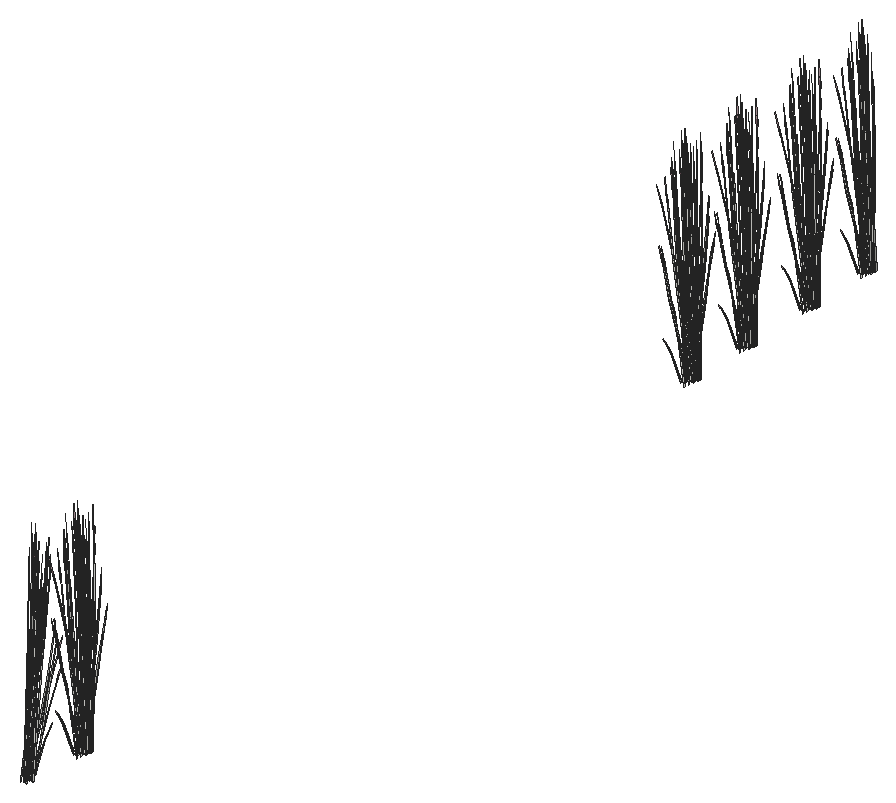
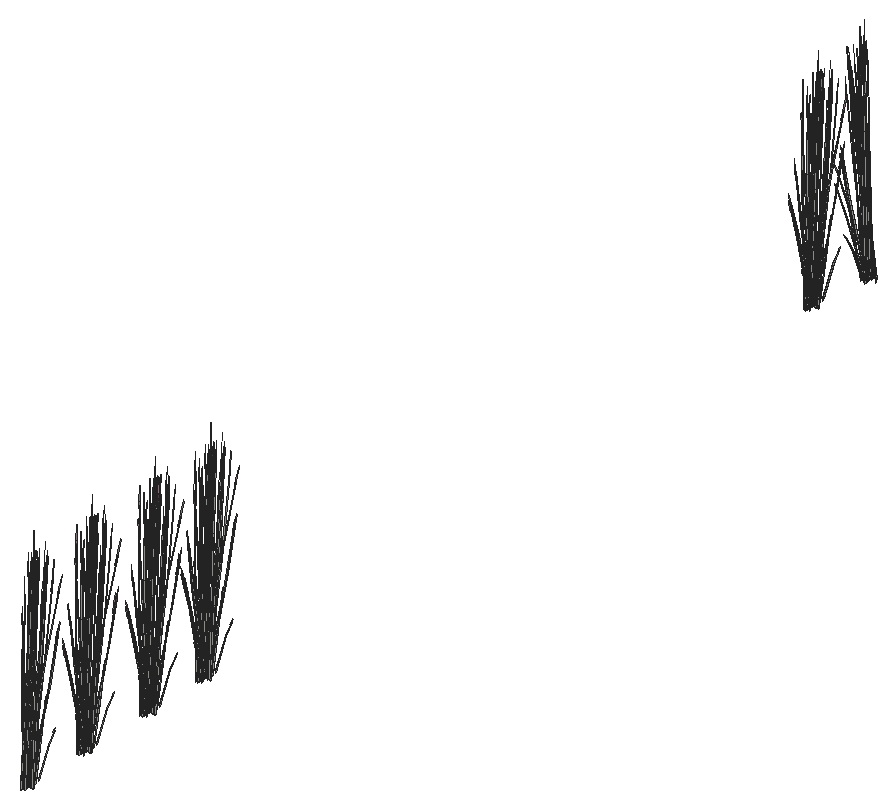
# SketchUp Ruby script. Lengths in inches.
U = 1.inch
M = Sketchup.active_model
def pt(a) = Geom::Point3d.new(a.map { |v| v * U })
def face(e, loops, mat)
  f = e.add_face(loops[0].map { |a| pt(a) })
  loops[1..].each { |l| e.add_face(l.map { |a| pt(a) }).erase! }
  f.material = f.back_material = mat if mat
  f
end
# faces: each face lists its corners as indices into pts; further lists are holes
def faces(e, pts, list, mat = nil) = list.each { |f| face(e, (f[0].is_a?(Array) ? f : [f]).map { |l| l.map { |i| pts[i] } }, mat) }
# xy, xz, yz: faces in a plane at the given z, y or x. An outline is a flat list of corners, or four numbers for a rectangle; further outlines are holes
def ring(l) = l.size == 4 ? [[l[0], l[1]], [l[2], l[1]], [l[2], l[3]], [l[0], l[3]]] : l.each_slice(2).to_a
def flat(e, list, mat, &to3) = list.each { |f| face(e, (f[0].is_a?(Array) ? f : [f]).map { |l| ring(l).map { |u, v| to3.(u, v) } }, mat) }
def xy(e, z, list, mat = nil) = flat(e, list, mat) { |x, y| [x, y, z] }
def xz(e, y, list, mat = nil) = flat(e, list, mat) { |x, z| [x, y, z] }
def yz(e, x, list, mat = nil) = flat(e, list, mat) { |y, z| [x, y, z] }
def lines(e, pts, list) = list.each { |a, b| e.add_line(pt(pts[a]), pt(pts[b])) }
# prism: a flat outline (further loops are holes) pulled along v
def prism(e, loops, v, mat = nil)
  f = face(e, loops, mat); d = Geom::Vector3d.new(v.map { |x| x * U })
  f.pushpull(f.normal.samedirection?(d) ? d.length : -d.length)
end
def box(e, o, s, mat = nil) = prism(e, [[o, [o[0] + s[0], o[1], o[2]], [o[0] + s[0], o[1] + s[1], o[2]], [o[0], o[1] + s[1], o[2]]]], [0, 0, s[2]], mat)
def at(x, y, z, deg = 0) = Geom::Transformation.translation(pt([x, y, z])) * Geom::Transformation.rotation(ORIGIN, Z_AXIS, deg.degrees)
def axes(o, x, y, z) = Geom::Transformation.new([*x, 0, *y, 0, *z, 0, *pt(o).to_a, 1])
def part(name) = M.definitions.add(name)
# library, detail: a bought-in or finely detailed component or shape, given as its bounding box
def library(name, o, s) = part(name).tap { |d| box(d.entities, o, s) }
def detail(e, o, s) = box(e.add_group.entities, o, s)
def put(e, d, t, mat = nil) = e.add_instance(d, t).tap { |i| i.material = mat if mat }
def group(e, t, mat = nil) = e.add_group.tap { |g| g.transformation = t; g.material = mat if mat }.entities
root = M.entities
M.materials.add("LightPink_Translucent").color = [144, 107, 117]
M.materials["LightPink_Translucent"].alpha = 0.75
c1 = part("blade")
p = [[2.15,0.21,22],[0,0.17,0],[0.09,0.45,0],[2.18,0.31,22],[2.29,0.31,22],[0.38,0.45,0],
  [2.48,0.24,33],[2.49,0.24,33],[2.48,0.22,33]]
faces(c1.entities,p,[[0,1,2,3],[4,5,2,3],[6,3,4,7],[8,0,3,6]])
c2 = part("seeds")
p = [[0.3,-0.1,1.38],[-0.01,-0.03,1.59],[-0.01,-0.03,0.03],[0.14,-0.07,-0.07],[0.29,-0.03,3],[0.15,0.01,3.11]]
faces(c2.entities,p,[[0,1,2,3],[1,0,4,5]],"LightPink_Translucent")
c3 = part("blade with seeds")
put(c3.entities,c1,at(0,0,0))
put(c3.entities,c2,axes([2.4,0.25,30.99],[1.5799,-0.05474,1.17369],[-0.12525,1.92788,0.29478],[-0.07173,-0.02425,1.56792]))
put(root,c3,axes([399.9,291.3,2.48],[-0.33032,-0.23318,0.49651],[0.19744,-0.41812,0],[0.07523,0.05311,1.57504]))
put(root,c3,axes([399.15,292.21,2.36],[-0.29264,0.42323,0.45755],[-0.34767,-0.3736,0.17955],[0.07055,-0.04224,1.58856]))
put(root,c3,axes([398.49,291.89,1.59],[-0.3474,0.18671,1.28929],[-0.11057,-0.53572,0.50096],[0.21332,0.00891,1.46642]))
put(root,c3,axes([399.42,292.03,2.62],[0.06809,-0.4162,0.1448],[0.33266,0.07225,-0.41347],[0.06054,0.04274,1.26744]))
put(root,c3,axes([399.28,292.14,2.72],[-0.21202,-0.39143,0.44739],[0.32115,-0.27564,-0.21531],[0.06861,0.04843,1.43643]))
put(root,c3,axes([399.39,292.16,2.67],[0.35635,-0.30962,-0.29095],[0.23697,0.43749,-0.50002],[0.08792,0.04443,1.59708]))
put(root,c3,axes([399.66,292.67,2.21],[0.39487,0,0],[0,0.48281,0],[0,0,1.78407]))
put(root,c3,axes([400.2,291.51,2.03],[0.08291,0.40636,-0.30978],[-0.32928,0.11539,0.30978],[0.06638,0.04686,1.38974]))
put(root,c3,axes([399.53,292.42,2.38],[-0.44609,-0.09826,0.49198],[0.09078,-0.55493,0.19306],[0.06519,0.05359,1.70813]))
put(root,c3,axes([399.61,293.74,2.18],[0.37054,-0.15823,-0.19198],[0.1302,0.45581,0.00008],[0.0409,-0.01749,1.73897]))
put(root,c3,axes([399.65,292.875,2.21],[0.24637,0.30123,0],[-0.24637,0.30123,0],[0,0,1.69266]))
put(root,c3,axes([399.65,292.52,2.72],[0.17124,-0.42022,0.44739],[0.35581,0.20224,-0.21531],[0,0.09687,1.43643]))
put(root,c3,axes([399.62,292.38,2.21],[0.21202,0.39143,-0.44739],[-0.32115,0.27564,0.21531],[0.06861,0.04843,1.43643]))
put(root,c3,axes([400.55,292.76,2.48],[0,-0.46636,0.49651],[0.39487,0,0],[0,0.10622,1.57504]))
put(root,c3,axes([399.8,292.62,2.62],[0.32884,-0.136,0.1448],[0.11516,0.38837,-0.41347],[0,0.08547,1.26744]))
put(root,c3,axes([399.5,293.98,2.2],[0.35581,0.20937,0],[-0.17124,0.43505,0],[0,0,1.74954]))
put(root,c3,axes([400.82,292.84,2.375],[0.44133,0,0],[0,0.52122,-0.51607],[0,0.11871,1.63711]))
put(root,c3,axes([399.6875,292.65,2.67],[0.39748,0.22252,-0.29095],[-0.19139,0.46966,-0.50002],[0.01249,0.11531,1.59708]))
put(root,c3,axes([400.55,293.18,2.03],[-0.24637,0.29097,-0.30978],[-0.24637,-0.29097,0.30978],[0,0.09372,1.38974]))
put(root,c3,axes([400.72,293.19,2.02],[0,0.46636,-0.49651],[-0.39487,0,0],[0,0.10622,1.57504]))
put(root,c3,axes([400.22,294.16,2.77],[-0.19872,-0.13409,1.1486],[0.2566,-0.13625,0.84392],[0.06921,0.11541,0.25299]))
put(root,c3,axes([399.84,293.13,2.09],[0.12941,0.42699,-0.69212],[-0.37279,0.15378,-0.18165],[0.0143,0.14459,1.52773]))
put(root,c3,axes([400.25,294.77,2.67],[-0.22633,-0.01463,1.0506],[0.14947,-0.31064,0.58006],[0.08941,0.11036,0.8241]))
put(root,c3,axes([399.51,294.02,2.59],[0.00623,-0.15459,1.43002],[0.29764,-0.17268,-0.30754],[0.09188,0.18503,0.61141]))
put(root,c3,axes([398.99,294.54,4.68],[0.34695,0.11691,-0.51099],[-0.11892,0.40083,-0.3958],[0.03181,0.16138,0.97773]))
put(root,c3,axes([399.19,293.71,3.875],[-0.08068,-0.14973,1.71376],[0.3728,-0.12606,0.13857],[0.08426,0.23506,0.73262]))
put(root,c3,axes([402.27,307.45,4.98],[-0.16845,-0.3792,-0.71045],[0.34676,-0.21133,0.08574],[-0.03939,-0.18322,1.00501]))
put(root,c3,axes([402.14,307.38,4.68],[-0.34695,-0.11691,-0.51099],[0.11892,-0.40083,-0.3958],[-0.03181,-0.16138,0.97773]))
put(root,c3,axes([401.0625,306.7,2.77],[0.18411,0.16231,1.1486],[-0.26813,0.09757,0.84392],[-0.05737,-0.12474,0.25299]))
put(root,c3,axes([401.49,308.88,2.1],[-0.14494,-0.47823,-0.69835],[0.41752,-0.17223,-0.18329],[-0.01602,-0.16194,1.54149]))
put(root,c3,axes([401.92,306.94,2.13],[-0.2439,0.26754,-0.03893],[-0.22348,-0.29302,-0.17649],[-0.01573,-0.08303,0.58215]))
put(root,c3,axes([402.23,310.11,3.33],[0.305,0.18805,1.51261],[-0.29879,0.40513,0.59816],[-0.13384,-0.24012,1.26806]))
put(root,c3,axes([400.63,308.8125,2.02],[0,-0.46636,-0.49651],[0.39487,0,0],[0,-0.10622,1.57504]))
put(root,c3,axes([400.8,308.82,2.03],[0.24637,-0.29097,-0.30978],[0.24637,0.29097,0.30978],[0,-0.09372,1.38974]))
put(root,c3,axes([401.67,309.35,2.67],[-0.39748,-0.22252,-0.29095],[0.19139,-0.46966,-0.50002],[-0.01249,-0.11531,1.59708]))
put(root,c3,axes([400.875,309.03,2.33],[-0.32829,0.39208,0.30756],[-0.32849,-0.38796,-0.36492],[-0.01146,-0.11134,1.64885]))
put(root,c3,axes([401.77,309.85,2.4375],[0.09355,-0.55261,-0.23429],[0.44354,0.09633,0.51271],[-0.0775,-0.07631,1.5644]))
put(root,c3,axes([400.8,309.24,2.48],[0,0.46636,0.49651],[-0.39487,0,0],[0,-0.10622,1.57504]))
put(root,c3,axes([401.73,309.62,2.21],[-0.21202,-0.39143,-0.44739],[0.32115,-0.27564,0.21531],[-0.06861,-0.04843,1.43643]))
put(root,c3,axes([401.7,309.48,2.72],[-0.17124,0.42022,0.44739],[-0.35581,-0.20224,-0.21531],[0,-0.09687,1.43643]))
put(root,c3,axes([402.44,309.53,2.3],[-0.32829,-0.4014,-0.06131],[0.32849,-0.40164,0],[-0.01146,-0.01402,1.75571]))
put(root,c3,axes([401.82,309.58,2.36],[0.44609,0.09826,0.45755],[-0.09078,0.55493,0.17955],[-0.06519,-0.05359,1.58856]))
put(root,c3,axes([401.58,310.47,2.47],[0.37926,-0.12378,0.17642],[0.09365,0.46065,0.35086],[-0.03382,-0.06712,1.60407]))
put(root,c3,axes([401.93,309.98,2.62],[-0.06809,0.4162,0.1448],[-0.33266,-0.07225,-0.41347],[-0.06054,-0.04274,1.26744]))
put(root,c3,axes([402.71,310.49,2.47],[0.10196,-0.46348,0.17642],[0.3731,0.13116,0.35086],[-0.06445,0.00226,1.60407]))
put(root,c3,axes([402.07,310.54,2.2],[-0.35581,-0.20937,0],[0.17124,-0.43505,0],[0,0,1.62707]))
put(root,c3,axes([402.36,309.98,2.46],[-0.34464,-0.37536,-0.25192],[0.29,-0.42149,0.5513],[-0.0928,0.04391,1.68216]))
put(root,c3,axes([401.45,310.7,2.48],[0.33032,0.23318,0.49651],[-0.19744,0.41812,0],[-0.07523,-0.05311,1.57504]))
put(root,c3,axes([402.53,309.67,2.72],[0.38326,-0.02879,0.44739],[0.03466,0.47788,-0.21531],[-0.06861,0.04843,1.43643]))
put(root,c3,axes([402.1875,309.9,2.21],[-0.38326,0.02879,-0.44739],[-0.03466,-0.47788,0.21531],[-0.06861,0.04843,1.43643]))
put(root,c3,axes([402.61,311.01,2.19],[-0.21791,-0.46895,-0.05142],[0.36918,-0.26061,0.51607],[-0.09097,0.04465,1.6363]))
put(root,c3,axes([402.53,309.875,2.62],[0.26075,0.2802,0.1448],[-0.2175,0.31612,-0.41347],[-0.06054,0.04274,1.26744]))
put(root,c3,axes([402.51,310.95,2.03],[-0.32928,-0.11539,-0.30978],[0.08291,-0.40636,0.30978],[-0.06638,0.04686,1.38974]))
put(root,c3,axes([402.46,309.77,2.67],[0.04113,0.53214,-0.29095],[-0.42835,0.03218,-0.50002],[-0.07543,0.07088,1.59708]))
put(root,c3,axes([402.2,310.18,2.06],[-0.23773,0.35053,-0.62353],[-0.29532,-0.31785,-0.16365],[-0.09526,0.08744,1.37633]))
put(root,c3,axes([402.59,311.14,2.02],[-0.33032,0.23318,-0.49651],[-0.19744,-0.41812,0],[-0.07523,0.05311,1.57504]))
put(root,c3,axes([402.89,311.0625,2.375],[0.22066,0.46731,0],[-0.36918,0.26061,-0.51607],[-0.08408,0.05936,1.63711]))
put(root,c3,axes([402.7,309.21,2.84],[-0.00964,-0.43909,1.41272],[0.43635,0.11382,0.59816],[-0.1032,0.24027,1.3335]))
put(root,c3,axes([400.98,310.91,4.53],[-0.23881,0.24554,-0.35414],[-0.22606,-0.28036,0.4572],[-0.0344,0.14245,0.87481]))
put(root,c3,axes([401.13,311.87,2.77],[-0.00913,-0.2773,1.1486],[0.22824,0.19778,0.84392],[-0.04489,0.13217,0.25299]))
put(root,c3,axes([401.21,310.8,5],[0.25266,0.31335,-0.5672],[-0.2669,0.27442,-0.43934],[-0.03844,0.15921,1.08528]))
put(root,c3,axes([400.9375,311.27,2.82],[0.32063,-0.08258,0.06507],[0.07371,0.33271,-0.86304],[-0.02033,0.16842,0.7736]))
put(root,c3,axes([401.13,310.65,5.34],[-0.00918,0.43138,-0.7886],[-0.38672,-0.02897,0.09517],[-0.04081,0.18275,1.11556]))
put(root,c3,axes([401.5,310.35,3.875],[-0.00864,-0.17899,1.71376],[0.37441,0.11874,0.13857],[-0.02316,0.25508,0.73262]))
put(root,c3,axes([401.01,311.26,3.36],[0.00775,-0.24075,1.54345],[0.34877,0.12716,0.21329],[-0.03022,0.25658,0.72882]))
put(root,c3,axes([402.27,517.89,4.98],[-0.16845,-0.3792,-0.71045],[0.34676,-0.21133,0.08574],[-0.03939,-0.18322,1.00501]))
put(root,c3,axes([402.14,517.8125,4.68],[-0.34695,-0.11691,-0.51099],[0.11892,-0.40083,-0.3958],[-0.03181,-0.16138,0.97773]))
put(root,c3,axes([401.0625,517.14,2.77],[0.18411,0.16231,1.1486],[-0.26813,0.09757,0.84392],[-0.05737,-0.12474,0.25299]))
put(root,c3,axes([401.49,519.3125,2.1],[-0.14494,-0.47823,-0.69835],[0.41752,-0.17223,-0.18329],[-0.01602,-0.16194,1.54149]))
put(root,c3,axes([401.92,517.375,2.13],[-0.2439,0.26754,-0.03893],[-0.22348,-0.29302,-0.17649],[-0.01573,-0.08303,0.58215]))
put(root,c3,axes([402.23,520.55,3.33],[0.305,0.18805,1.51261],[-0.29879,0.40513,0.59816],[-0.13384,-0.24012,1.26806]))
put(root,c3,axes([400.63,519.25,2.02],[0,-0.46636,-0.49651],[0.39487,0,0],[0,-0.10622,1.57504]))
put(root,c3,axes([400.8,519.26,2.03],[0.24637,-0.29097,-0.30978],[0.24637,0.29097,0.30978],[0,-0.09372,1.38974]))
put(root,c3,axes([401.67,519.79,2.67],[-0.39748,-0.22252,-0.29095],[0.19139,-0.46966,-0.50002],[-0.01249,-0.11531,1.59708]))
put(root,c3,axes([400.875,519.46,2.33],[-0.32829,0.39208,0.30756],[-0.32849,-0.38796,-0.36492],[-0.01146,-0.11134,1.64885]))
put(root,c3,axes([401.77,520.28,2.4375],[0.09355,-0.55261,-0.23429],[0.44354,0.09633,0.51271],[-0.0775,-0.07631,1.5644]))
put(root,c3,axes([400.8,519.68,2.48],[0,0.46636,0.49651],[-0.39487,0,0],[0,-0.10622,1.57504]))
put(root,c3,axes([401.73,520.06,2.21],[-0.21202,-0.39143,-0.44739],[0.32115,-0.27564,0.21531],[-0.06861,-0.04843,1.43643]))
put(root,c3,axes([401.7,519.91,2.72],[-0.17124,0.42022,0.44739],[-0.35581,-0.20224,-0.21531],[0,-0.09687,1.43643]))
put(root,c3,axes([402.44,519.97,2.3],[-0.32829,-0.4014,-0.06131],[0.32849,-0.40164,0],[-0.01146,-0.01402,1.75571]))
put(root,c3,axes([401.82,520.02,2.36],[0.44609,0.09826,0.45755],[-0.09078,0.55493,0.17955],[-0.06519,-0.05359,1.58856]))
put(root,c3,axes([401.58,520.9,2.47],[0.37926,-0.12378,0.17642],[0.09365,0.46065,0.35086],[-0.03382,-0.06712,1.60407]))
put(root,c3,axes([401.93,520.41,2.62],[-0.06809,0.4162,0.1448],[-0.33266,-0.07225,-0.41347],[-0.06054,-0.04274,1.26744]))
put(root,c3,axes([402.71,520.93,2.47],[0.10196,-0.46348,0.17642],[0.3731,0.13116,0.35086],[-0.06445,0.00226,1.60407]))
put(root,c3,axes([402.07,520.97,2.2],[-0.35581,-0.20937,0],[0.17124,-0.43505,0],[0,0,1.62707]))
put(root,c3,axes([402.36,520.42,2.46],[-0.34464,-0.37536,-0.25192],[0.29,-0.42149,0.5513],[-0.0928,0.04391,1.68216]))
put(root,c3,axes([401.45,521.14,2.48],[0.33032,0.23318,0.49651],[-0.19744,0.41812,0],[-0.07523,-0.05311,1.57504]))
put(root,c3,axes([402.53,520.11,2.72],[0.38326,-0.02879,0.44739],[0.03466,0.47788,-0.21531],[-0.06861,0.04843,1.43643]))
put(root,c3,axes([402.1875,520.34,2.21],[-0.38326,0.02879,-0.44739],[-0.03466,-0.47788,0.21531],[-0.06861,0.04843,1.43643]))
put(root,c3,axes([402.61,521.45,2.19],[-0.21791,-0.46895,-0.05142],[0.36918,-0.26061,0.51607],[-0.09097,0.04465,1.6363]))
put(root,c3,axes([402.53,520.3125,2.62],[0.26075,0.2802,0.1448],[-0.2175,0.31612,-0.41347],[-0.06054,0.04274,1.26744]))
put(root,c3,axes([402.51,521.39,2.03],[-0.32928,-0.11539,-0.30978],[0.08291,-0.40636,0.30978],[-0.06638,0.04686,1.38974]))
put(root,c3,axes([402.46,520.21,2.67],[0.04113,0.53214,-0.29095],[-0.42835,0.03218,-0.50002],[-0.07543,0.07088,1.59708]))
put(root,c3,axes([402.2,520.61,2.06],[-0.23773,0.35053,-0.62353],[-0.29532,-0.31785,-0.16365],[-0.09526,0.08744,1.37633]))
put(root,c3,axes([402.59,521.57,2.02],[-0.33032,0.23318,-0.49651],[-0.19744,-0.41812,0],[-0.07523,0.05311,1.57504]))
put(root,c3,axes([402.89,521.5,2.375],[0.22066,0.46731,0],[-0.36918,0.26061,-0.51607],[-0.08408,0.05936,1.63711]))
put(root,c3,axes([402.7,519.65,2.84],[-0.00964,-0.43909,1.41272],[0.43635,0.11382,0.59816],[-0.1032,0.24027,1.3335]))
put(root,c3,axes([400.98,521.35,4.53],[-0.23881,0.24554,-0.35414],[-0.22606,-0.28036,0.4572],[-0.0344,0.14245,0.87481]))
put(root,c3,axes([401.13,522.3,2.77],[-0.00913,-0.2773,1.1486],[0.22824,0.19778,0.84392],[-0.04489,0.13217,0.25299]))
put(root,c3,axes([401.21,521.23,5],[0.25266,0.31335,-0.5672],[-0.2669,0.27442,-0.43934],[-0.03844,0.15921,1.08528]))
put(root,c3,axes([400.9375,521.7,2.82],[0.32063,-0.08258,0.06507],[0.07371,0.33271,-0.86304],[-0.02033,0.16842,0.7736]))
put(root,c3,axes([401.13,521.09,5.34],[-0.00918,0.43138,-0.7886],[-0.38672,-0.02897,0.09517],[-0.04081,0.18275,1.11556]))
put(root,c3,axes([401.5,520.78,3.875],[-0.00864,-0.17899,1.71376],[0.37441,0.11874,0.13857],[-0.02316,0.25508,0.73262]))
put(root,c3,axes([401.01,521.7,3.36],[0.00775,-0.24075,1.54345],[0.34877,0.12716,0.21329],[-0.03022,0.25658,0.72882]))
put(root,c3,axes([402.27,537.12,4.98],[-0.16845,-0.3792,-0.71045],[0.34676,-0.21133,0.08574],[-0.03939,-0.18322,1.00501]))
put(root,c3,axes([402.14,537.04,4.68],[-0.34695,-0.11691,-0.51099],[0.11892,-0.40083,-0.3958],[-0.03181,-0.16138,0.97773]))
put(root,c3,axes([401.0625,536.37,2.77],[0.18411,0.16231,1.1486],[-0.26813,0.09757,0.84392],[-0.05737,-0.12474,0.25299]))
put(root,c3,axes([401.49,538.54,2.1],[-0.14494,-0.47823,-0.69835],[0.41752,-0.17223,-0.18329],[-0.01602,-0.16194,1.54149]))
put(root,c3,axes([401.92,536.6,2.13],[-0.2439,0.26754,-0.03893],[-0.22348,-0.29302,-0.17649],[-0.01573,-0.08303,0.58215]))
put(root,c3,axes([402.23,539.78,3.33],[0.305,0.18805,1.51261],[-0.29879,0.40513,0.59816],[-0.13384,-0.24012,1.26806]))
put(root,c3,axes([400.63,538.48,2.02],[0,-0.46636,-0.49651],[0.39487,0,0],[0,-0.10622,1.57504]))
put(root,c3,axes([400.8,538.49,2.03],[0.24637,-0.29097,-0.30978],[0.24637,0.29097,0.30978],[0,-0.09372,1.38974]))
put(root,c3,axes([401.67,539.02,2.67],[-0.39748,-0.22252,-0.29095],[0.19139,-0.46966,-0.50002],[-0.01249,-0.11531,1.59708]))
put(root,c3,axes([400.875,538.69,2.33],[-0.32829,0.39208,0.30756],[-0.32849,-0.38796,-0.36492],[-0.01146,-0.11134,1.64885]))
put(root,c3,axes([401.77,539.51,2.4375],[0.09355,-0.55261,-0.23429],[0.44354,0.09633,0.51271],[-0.0775,-0.07631,1.5644]))
put(root,c3,axes([400.8,538.91,2.48],[0,0.46636,0.49651],[-0.39487,0,0],[0,-0.10622,1.57504]))
put(root,c3,axes([401.73,539.28,2.21],[-0.21202,-0.39143,-0.44739],[0.32115,-0.27564,0.21531],[-0.06861,-0.04843,1.43643]))
put(root,c3,axes([401.7,539.14,2.72],[-0.17124,0.42022,0.44739],[-0.35581,-0.20224,-0.21531],[0,-0.09687,1.43643]))
put(root,c3,axes([402.44,539.19,2.3],[-0.32829,-0.4014,-0.06131],[0.32849,-0.40164,0],[-0.01146,-0.01402,1.75571]))
put(root,c3,axes([401.82,539.24,2.36],[0.44609,0.09826,0.45755],[-0.09078,0.55493,0.17955],[-0.06519,-0.05359,1.58856]))
put(root,c3,axes([401.58,540.13,2.47],[0.37926,-0.12378,0.17642],[0.09365,0.46065,0.35086],[-0.03382,-0.06712,1.60407]))
put(root,c3,axes([401.93,539.64,2.62],[-0.06809,0.4162,0.1448],[-0.33266,-0.07225,-0.41347],[-0.06054,-0.04274,1.26744]))
put(root,c3,axes([402.71,540.15,2.47],[0.10196,-0.46348,0.17642],[0.3731,0.13116,0.35086],[-0.06445,0.00226,1.60407]))
put(root,c3,axes([402.07,540.2,2.2],[-0.35581,-0.20937,0],[0.17124,-0.43505,0],[0,0,1.62707]))
put(root,c3,axes([402.36,539.65,2.46],[-0.34464,-0.37536,-0.25192],[0.29,-0.42149,0.5513],[-0.0928,0.04391,1.68216]))
put(root,c3,axes([401.45,540.36,2.48],[0.33032,0.23318,0.49651],[-0.19744,0.41812,0],[-0.07523,-0.05311,1.57504]))
put(root,c3,axes([402.53,539.33,2.72],[0.38326,-0.02879,0.44739],[0.03466,0.47788,-0.21531],[-0.06861,0.04843,1.43643]))
put(root,c3,axes([402.1875,539.57,2.21],[-0.38326,0.02879,-0.44739],[-0.03466,-0.47788,0.21531],[-0.06861,0.04843,1.43643]))
put(root,c3,axes([402.61,540.67,2.19],[-0.21791,-0.46895,-0.05142],[0.36918,-0.26061,0.51607],[-0.09097,0.04465,1.6363]))
put(root,c3,axes([402.53,539.54,2.62],[0.26075,0.2802,0.1448],[-0.2175,0.31612,-0.41347],[-0.06054,0.04274,1.26744]))
put(root,c3,axes([402.51,540.61,2.03],[-0.32928,-0.11539,-0.30978],[0.08291,-0.40636,0.30978],[-0.06638,0.04686,1.38974]))
put(root,c3,axes([402.46,539.4375,2.67],[0.04113,0.53214,-0.29095],[-0.42835,0.03218,-0.50002],[-0.07543,0.07088,1.59708]))
put(root,c3,axes([402.2,539.84,2.06],[-0.23773,0.35053,-0.62353],[-0.29532,-0.31785,-0.16365],[-0.09526,0.08744,1.37633]))
put(root,c3,axes([402.59,540.8,2.02],[-0.33032,0.23318,-0.49651],[-0.19744,-0.41812,0],[-0.07523,0.05311,1.57504]))
put(root,c3,axes([402.89,540.73,2.375],[0.22066,0.46731,0],[-0.36918,0.26061,-0.51607],[-0.08408,0.05936,1.63711]))
put(root,c3,axes([402.7,538.875,2.84],[-0.00964,-0.43909,1.41272],[0.43635,0.11382,0.59816],[-0.1032,0.24027,1.3335]))
put(root,c3,axes([400.98,540.58,4.53],[-0.23881,0.24554,-0.35414],[-0.22606,-0.28036,0.4572],[-0.0344,0.14245,0.87481]))
put(root,c3,axes([401.13,541.53,2.77],[-0.00913,-0.2773,1.1486],[0.22824,0.19778,0.84392],[-0.04489,0.13217,0.25299]))
put(root,c3,axes([401.21,540.46,5],[0.25266,0.31335,-0.5672],[-0.2669,0.27442,-0.43934],[-0.03844,0.15921,1.08528]))
put(root,c3,axes([400.9375,540.93,2.82],[0.32063,-0.08258,0.06507],[0.07371,0.33271,-0.86304],[-0.02033,0.16842,0.7736]))
put(root,c3,axes([401.13,540.32,5.34],[-0.00918,0.43138,-0.7886],[-0.38672,-0.02897,0.09517],[-0.04081,0.18275,1.11556]))
put(root,c3,axes([401.5,540.01,3.875],[-0.00864,-0.17899,1.71376],[0.37441,0.11874,0.13857],[-0.02316,0.25508,0.73262]))
put(root,c3,axes([401.01,540.93,3.36],[0.00775,-0.24075,1.54345],[0.34877,0.12716,0.21329],[-0.03022,0.25658,0.72882]))
put(root,c3,axes([402.27,558.96,4.98],[-0.16845,-0.3792,-0.71045],[0.34676,-0.21133,0.08574],[-0.03939,-0.18322,1.00501]))
put(root,c3,axes([402.14,558.89,4.68],[-0.34695,-0.11691,-0.51099],[0.11892,-0.40083,-0.3958],[-0.03181,-0.16138,0.97773]))
put(root,c3,axes([401.0625,558.21,2.77],[0.18411,0.16231,1.1486],[-0.26813,0.09757,0.84392],[-0.05737,-0.12474,0.25299]))
put(root,c3,axes([401.49,560.39,2.1],[-0.14494,-0.47823,-0.69835],[0.41752,-0.17223,-0.18329],[-0.01602,-0.16194,1.54149]))
put(root,c3,axes([401.92,558.45,2.13],[-0.2439,0.26754,-0.03893],[-0.22348,-0.29302,-0.17649],[-0.01573,-0.08303,0.58215]))
put(root,c3,axes([402.23,561.62,3.33],[0.305,0.18805,1.51261],[-0.29879,0.40513,0.59816],[-0.13384,-0.24012,1.26806]))
put(root,c3,axes([400.63,560.32,2.02],[0,-0.46636,-0.49651],[0.39487,0,0],[0,-0.10622,1.57504]))
put(root,c3,axes([400.8,560.33,2.03],[0.24637,-0.29097,-0.30978],[0.24637,0.29097,0.30978],[0,-0.09372,1.38974]))
put(root,c3,axes([401.67,560.86,2.67],[-0.39748,-0.22252,-0.29095],[0.19139,-0.46966,-0.50002],[-0.01249,-0.11531,1.59708]))
put(root,c3,axes([400.875,560.54,2.33],[-0.32829,0.39208,0.30756],[-0.32849,-0.38796,-0.36492],[-0.01146,-0.11134,1.64885]))
put(root,c3,axes([401.77,561.35,2.4375],[0.09355,-0.55261,-0.23429],[0.44354,0.09633,0.51271],[-0.0775,-0.07631,1.5644]))
put(root,c3,axes([400.8,560.75,2.48],[0,0.46636,0.49651],[-0.39487,0,0],[0,-0.10622,1.57504]))
put(root,c3,axes([401.73,561.13,2.21],[-0.21202,-0.39143,-0.44739],[0.32115,-0.27564,0.21531],[-0.06861,-0.04843,1.43643]))
put(root,c3,axes([401.7,560.99,2.72],[-0.17124,0.42022,0.44739],[-0.35581,-0.20224,-0.21531],[0,-0.09687,1.43643]))
put(root,c3,axes([402.44,561.04,2.3],[-0.32829,-0.4014,-0.06131],[0.32849,-0.40164,0],[-0.01146,-0.01402,1.75571]))
put(root,c3,axes([401.82,561.09,2.36],[0.44609,0.09826,0.45755],[-0.09078,0.55493,0.17955],[-0.06519,-0.05359,1.58856]))
put(root,c3,axes([401.58,561.97,2.47],[0.37926,-0.12378,0.17642],[0.09365,0.46065,0.35086],[-0.03382,-0.06712,1.60407]))
put(root,c3,axes([401.93,561.48,2.62],[-0.06809,0.4162,0.1448],[-0.33266,-0.07225,-0.41347],[-0.06054,-0.04274,1.26744]))
put(root,c3,axes([402.71,562,2.47],[0.10196,-0.46348,0.17642],[0.3731,0.13116,0.35086],[-0.06445,0.00226,1.60407]))
put(root,c3,axes([402.07,562.05,2.2],[-0.35581,-0.20937,0],[0.17124,-0.43505,0],[0,0,1.62707]))
put(root,c3,axes([402.36,561.49,2.46],[-0.34464,-0.37536,-0.25192],[0.29,-0.42149,0.5513],[-0.0928,0.04391,1.68216]))
put(root,c3,axes([401.45,562.21,2.48],[0.33032,0.23318,0.49651],[-0.19744,0.41812,0],[-0.07523,-0.05311,1.57504]))
put(root,c3,axes([402.53,561.18,2.72],[0.38326,-0.02879,0.44739],[0.03466,0.47788,-0.21531],[-0.06861,0.04843,1.43643]))
put(root,c3,axes([402.1875,561.41,2.21],[-0.38326,0.02879,-0.44739],[-0.03466,-0.47788,0.21531],[-0.06861,0.04843,1.43643]))
put(root,c3,axes([402.61,562.52,2.19],[-0.21791,-0.46895,-0.05142],[0.36918,-0.26061,0.51607],[-0.09097,0.04465,1.6363]))
put(root,c3,axes([402.53,561.38,2.62],[0.26075,0.2802,0.1448],[-0.2175,0.31612,-0.41347],[-0.06054,0.04274,1.26744]))
put(root,c3,axes([402.51,562.46,2.03],[-0.32928,-0.11539,-0.30978],[0.08291,-0.40636,0.30978],[-0.06638,0.04686,1.38974]))
put(root,c3,axes([402.46,561.28,2.67],[0.04113,0.53214,-0.29095],[-0.42835,0.03218,-0.50002],[-0.07543,0.07088,1.59708]))
put(root,c3,axes([402.2,561.6875,2.06],[-0.23773,0.35053,-0.62353],[-0.29532,-0.31785,-0.16365],[-0.09526,0.08744,1.37633]))
put(root,c3,axes([402.59,562.64,2.02],[-0.33032,0.23318,-0.49651],[-0.19744,-0.41812,0],[-0.07523,0.05311,1.57504]))
put(root,c3,axes([402.89,562.57,2.375],[0.22066,0.46731,0],[-0.36918,0.26061,-0.51607],[-0.08408,0.05936,1.63711]))
put(root,c3,axes([402.7,560.72,2.84],[-0.00964,-0.43909,1.41272],[0.43635,0.11382,0.59816],[-0.1032,0.24027,1.3335]))
put(root,c3,axes([400.98,562.42,4.53],[-0.23881,0.24554,-0.35414],[-0.22606,-0.28036,0.4572],[-0.0344,0.14245,0.87481]))
put(root,c3,axes([401.13,563.375,2.77],[-0.00913,-0.2773,1.1486],[0.22824,0.19778,0.84392],[-0.04489,0.13217,0.25299]))
put(root,c3,axes([401.21,562.31,5],[0.25266,0.31335,-0.5672],[-0.2669,0.27442,-0.43934],[-0.03844,0.15921,1.08528]))
put(root,c3,axes([400.9375,562.78,2.82],[0.32063,-0.08258,0.06507],[0.07371,0.33271,-0.86304],[-0.02033,0.16842,0.7736]))
put(root,c3,axes([401.13,562.16,5.34],[-0.00918,0.43138,-0.7886],[-0.38672,-0.02897,0.09517],[-0.04081,0.18275,1.11556]))
put(root,c3,axes([401.5,561.86,3.875],[-0.00864,-0.17899,1.71376],[0.37441,0.11874,0.13857],[-0.02316,0.25508,0.73262]))
put(root,c3,axes([401.01,562.77,3.36],[0.00775,-0.24075,1.54345],[0.34877,0.12716,0.21329],[-0.03022,0.25658,0.72882]))
put(root,c3,axes([402.27,579.23,4.98],[-0.16845,-0.3792,-0.71045],[0.34676,-0.21133,0.08574],[-0.03939,-0.18322,1.00501]))
put(root,c3,axes([402.14,579.15,4.68],[-0.34695,-0.11691,-0.51099],[0.11892,-0.40083,-0.3958],[-0.03181,-0.16138,0.97773]))
put(root,c3,axes([401.0625,578.48,2.77],[0.18411,0.16231,1.1486],[-0.26813,0.09757,0.84392],[-0.05737,-0.12474,0.25299]))
put(root,c3,axes([401.49,580.65,2.1],[-0.14494,-0.47823,-0.69835],[0.41752,-0.17223,-0.18329],[-0.01602,-0.16194,1.54149]))
put(root,c3,axes([401.92,578.72,2.13],[-0.2439,0.26754,-0.03893],[-0.22348,-0.29302,-0.17649],[-0.01573,-0.08303,0.58215]))
put(root,c3,axes([402.23,581.89,3.33],[0.305,0.18805,1.51261],[-0.29879,0.40513,0.59816],[-0.13384,-0.24012,1.26806]))
put(root,c3,axes([400.63,580.59,2.02],[0,-0.46636,-0.49651],[0.39487,0,0],[0,-0.10622,1.57504]))
put(root,c3,axes([400.8,580.6,2.03],[0.24637,-0.29097,-0.30978],[0.24637,0.29097,0.30978],[0,-0.09372,1.38974]))
put(root,c3,axes([401.67,581.13,2.67],[-0.39748,-0.22252,-0.29095],[0.19139,-0.46966,-0.50002],[-0.01249,-0.11531,1.59708]))
put(root,c3,axes([400.875,580.8,2.33],[-0.32829,0.39208,0.30756],[-0.32849,-0.38796,-0.36492],[-0.01146,-0.11134,1.64885]))
put(root,c3,axes([401.77,581.62,2.4375],[0.09355,-0.55261,-0.23429],[0.44354,0.09633,0.51271],[-0.0775,-0.07631,1.5644]))
put(root,c3,axes([400.8,581.02,2.48],[0,0.46636,0.49651],[-0.39487,0,0],[0,-0.10622,1.57504]))
put(root,c3,axes([401.73,581.4,2.21],[-0.21202,-0.39143,-0.44739],[0.32115,-0.27564,0.21531],[-0.06861,-0.04843,1.43643]))
put(root,c3,axes([401.7,581.26,2.72],[-0.17124,0.42022,0.44739],[-0.35581,-0.20224,-0.21531],[0,-0.09687,1.43643]))
put(root,c3,axes([402.44,581.31,2.3],[-0.32829,-0.4014,-0.06131],[0.32849,-0.40164,0],[-0.01146,-0.01402,1.75571]))
put(root,c3,axes([401.82,581.36,2.36],[0.44609,0.09826,0.45755],[-0.09078,0.55493,0.17955],[-0.06519,-0.05359,1.58856]))
put(root,c3,axes([401.58,582.24,2.47],[0.37926,-0.12378,0.17642],[0.09365,0.46065,0.35086],[-0.03382,-0.06712,1.60407]))
put(root,c3,axes([401.93,581.75,2.62],[-0.06809,0.4162,0.1448],[-0.33266,-0.07225,-0.41347],[-0.06054,-0.04274,1.26744]))
put(root,c3,axes([402.71,582.27,2.47],[0.10196,-0.46348,0.17642],[0.3731,0.13116,0.35086],[-0.06445,0.00226,1.60407]))
put(root,c3,axes([402.07,582.32,2.2],[-0.35581,-0.20937,0],[0.17124,-0.43505,0],[0,0,1.62707]))
put(root,c3,axes([402.36,581.76,2.46],[-0.34464,-0.37536,-0.25192],[0.29,-0.42149,0.5513],[-0.0928,0.04391,1.68216]))
put(root,c3,axes([401.45,582.48,2.48],[0.33032,0.23318,0.49651],[-0.19744,0.41812,0],[-0.07523,-0.05311,1.57504]))
put(root,c3,axes([402.53,581.45,2.72],[0.38326,-0.02879,0.44739],[0.03466,0.47788,-0.21531],[-0.06861,0.04843,1.43643]))
put(root,c3,axes([402.1875,581.68,2.21],[-0.38326,0.02879,-0.44739],[-0.03466,-0.47788,0.21531],[-0.06861,0.04843,1.43643]))
put(root,c3,axes([402.61,582.79,2.19],[-0.21791,-0.46895,-0.05142],[0.36918,-0.26061,0.51607],[-0.09097,0.04465,1.6363]))
put(root,c3,axes([402.53,581.65,2.62],[0.26075,0.2802,0.1448],[-0.2175,0.31612,-0.41347],[-0.06054,0.04274,1.26744]))
put(root,c3,axes([402.51,582.73,2.03],[-0.32928,-0.11539,-0.30978],[0.08291,-0.40636,0.30978],[-0.06638,0.04686,1.38974]))
